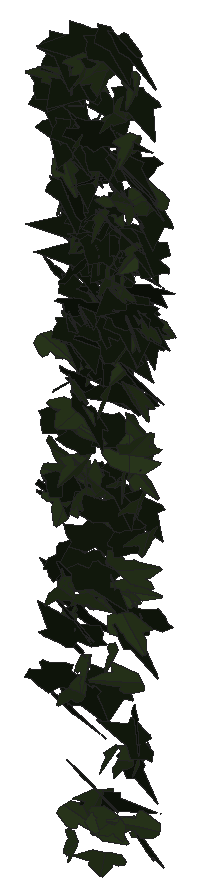
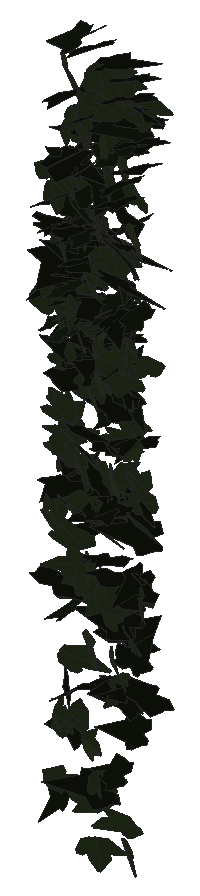
# SketchUp Ruby script. Lengths in millimetres.
U = 1.mm
M = Sketchup.active_model
def pt(a) = Geom::Point3d.new(a.map { |v| v * U })
def face(e, loops, mat)
  f = e.add_face(loops[0].map { |a| pt(a) })
  loops[1..].each { |l| e.add_face(l.map { |a| pt(a) }).erase! }
  f.material = f.back_material = mat if mat
  f
end
# faces: each face lists its corners as indices into pts; further lists are holes
def faces(e, pts, list, mat = nil) = list.each { |f| face(e, (f[0].is_a?(Array) ? f : [f]).map { |l| l.map { |i| pts[i] } }, mat) }
# xy, xz, yz: faces in a plane at the given z, y or x. An outline is a flat list of corners, or four numbers for a rectangle; further outlines are holes
def ring(l) = l.size == 4 ? [[l[0], l[1]], [l[2], l[1]], [l[2], l[3]], [l[0], l[3]]] : l.each_slice(2).to_a
def flat(e, list, mat, &to3) = list.each { |f| face(e, (f[0].is_a?(Array) ? f : [f]).map { |l| ring(l).map { |u, v| to3.(u, v) } }, mat) }
def xy(e, z, list, mat = nil) = flat(e, list, mat) { |x, y| [x, y, z] }
def xz(e, y, list, mat = nil) = flat(e, list, mat) { |x, z| [x, y, z] }
def yz(e, x, list, mat = nil) = flat(e, list, mat) { |y, z| [x, y, z] }
def lines(e, pts, list) = list.each { |a, b| e.add_line(pt(pts[a]), pt(pts[b])) }
# prism: a flat outline (further loops are holes) pulled along v
def prism(e, loops, v, mat = nil)
  f = face(e, loops, mat); d = Geom::Vector3d.new(v.map { |x| x * U })
  f.pushpull(f.normal.samedirection?(d) ? d.length : -d.length)
end
def box(e, o, s, mat = nil) = prism(e, [[o, [o[0] + s[0], o[1], o[2]], [o[0] + s[0], o[1] + s[1], o[2]], [o[0], o[1] + s[1], o[2]]]], [0, 0, s[2]], mat)
def at(x, y, z, deg = 0) = Geom::Transformation.translation(pt([x, y, z])) * Geom::Transformation.rotation(ORIGIN, Z_AXIS, deg.degrees)
def axes(o, x, y, z) = Geom::Transformation.new([*x, 0, *y, 0, *z, 0, *pt(o).to_a, 1])
def part(name) = M.definitions.add(name)
# library, detail: a bought-in or finely detailed component or shape, given as its bounding box
def library(name, o, s) = part(name).tap { |d| box(d.entities, o, s) }
def detail(e, o, s) = box(e.add_group.entities, o, s)
def put(e, d, t, mat = nil) = e.add_instance(d, t).tap { |i| i.material = mat if mat }
def group(e, t, mat = nil) = e.add_group.tap { |g| g.transformation = t; g.material = mat if mat }.entities
root = M.entities
M.materials.add("efeu1").color = [18, 25, 13]
M.materials.add("efeu2").color = [43, 57, 29]
c1 = part("ivyleaf_9")
p = [[39.1,54.8,31.7],[34.5,51.8,30.2],[-5.3,25.2,17.3],[-17.9,28.3,20.9],[-21.6,21.7,17],[-20.2,4.3,5.3],
  [-22.9,-0.3,2.5],[-17.1,-4,-0.6],[-2,-2.1,-1.2],[-0.7,-15.4,-10.1],[16.6,-22.3,-16.7],[21.1,-15.1,-12.5],
  [32.7,-10.7,-11],[46.1,-1.8,-6.6],[30.8,11.2,3.8]]
faces(c1.entities,p,[[0,1,2,3,4,5,6,7,8,9,10,11,12,13,14]],"efeu1")
c2 = part("ivyleaf_10")
p = [[0,12.8,-0.8],[-1.5,51.3,-10.9],[-4.9,51,-11.6],[-13.6,26.5,-7.3],[-13.2,15.9,-4.6],[-21.1,19.3,-7.2],
  [-29.5,16.3,-8.3],[-29.2,8.3,-6.2],[-19.7,-9.8,0.5],[-7.6,-13,4],[1,-12.2,5.8],[-0.4,51.1,-11.1],
  [-1.5,51.1,-10.9],[1,-12.4,5.9],[16.9,-12.4,3.5],[35.1,9.1,-5.1],[35,12.9,-6.1],[20.5,16.4,-4.9],
  [15.8,15,-3.8],[15.3,27.6,-7.1],[12.8,31.3,-7.8]]
faces(c2.entities,p,[[0,1,2,3,4,5,6,7,8,9,10],[11,12,0,13,14,15,16,17,18,19,20]],"efeu2")
put(root,c1,axes([2108.3,967.1,644.8],[1.00488,-0.20839,-0.71065],[1.27223,-0.24155,0.56748],[-0.60667,-0.85174,0.01293]))
put(root,c2,axes([2115.5,961.4,1563.5],[-0.34583,0.64404,-0.48709],[0.15743,-0.4818,-0.6679],[-1.52874,-0.19531,0.04141]))
put(root,c2,axes([2112.9,945,696],[-0.29657,-0.59672,-0.59249],[0.40636,0.55475,-0.61487],[1.54797,-0.25996,0.0479]))
put(root,c2,axes([2130.7,968.5,900.1],[-0.13701,-0.55796,0.633],[0.07222,-0.63679,-0.55699],[1.6043,-0.01898,0.07913]))
put(root,c1,axes([2165,954.3,739.4],[0.05238,-0.56762,-0.51326],[0.37061,0.50188,-0.54459],[1.4085,-0.11095,0.16239]))
put(root,c2,axes([2176.4,947.7,1276],[0.79385,-0.52482,-0.47962],[-0.14077,0.52102,-0.63445],[1.34577,0.36409,0.21656]))
put(root,c1,axes([2140.5,961.2,1130.8],[-0.37396,-0.7341,-0.27689],[0.2109,0.25662,-0.75898],[1.47825,-0.22232,0.03824]))
put(root,c1,axes([2131.3,969.4,1536.4],[-1.26194,-0.47663,0.15068],[-0.01345,-0.24134,-0.7945],[0.95127,-0.6357,0.18866]))
put(root,c2,axes([2101.8,955.2,1545.3],[-1.15192,-0.56127,0.00643],[-0.00965,-0.00399,-0.82544],[1.06823,-0.60528,-0.00052]))
put(root,c1,axes([2146,969.2,995.5],[0.23611,-0.7653,0.36632],[0.0902,-0.36339,-0.77522],[1.61226,0.13241,-0.01027]))
put(root,c1,axes([2132.3,959.9,611.1],[0.74877,0.01244,0.76483],[-1.44263,0.12186,0.38793],[-0.19554,-0.85142,0.06669]))
put(root,c1,axes([2206.7,969.2,886.7],[0.10131,-0.80719,0.28495],[0.02782,-0.2846,-0.80894],[1.62892,0.05506,-0.00391]))
put(root,c1,axes([2158.5,952,1181.7],[0.48377,0.56591,-0.44058],[-0.55888,-0.34433,-0.6117],[-1.2453,0.37437,0.10337]))
put(root,c2,axes([2216.6,949.5,1442.1],[0.30113,-0.68342,-0.44499],[-0.00794,0.4526,-0.6966],[1.55208,0.13491,0.08277]))
put(root,c2,axes([2106.2,963.3,1390.3],[0.94252,-0.3055,0.55505],[0.96578,-0.23056,-0.57966],[0.72199,0.70723,0.05079]))
put(root,c1,axes([2201.5,949.6,838.4],[-0.80201,-0.07863,0.75132],[1.42849,0.05368,0.4266],[-0.16255,0.85975,0.04208]))
put(root,c2,axes([2133.2,957.9,993.3],[1.43151,-0.13805,-0.25891],[-0.48275,0.0522,-0.7647],[0.28072,0.79376,0.00526]))
put(root,c2,axes([2214.5,944.6,1521.6],[-0.1793,-0.63096,-0.69188],[0.24221,0.68029,-0.63772],[1.76559,-0.1574,0.01722]))
put(root,c2,axes([2199.9,956.8,337.1],[1.22763,-0.3477,-0.28676],[-0.47961,0.13685,-0.73278],[0.71115,0.69251,0.00083]))
put(root,c2,axes([2151.9,963.7,1580.9],[-0.42301,-0.77281,0.28209],[0.02369,-0.29533,-0.79928],[1.56556,-0.20434,0.08831]))
put(root,c2,axes([2241.9,957.1,1149],[-0.98131,0.58056,0.05581],[0.07125,-0.0414,0.77647],[1.10772,0.51697,-0.0005]))
put(root,c2,axes([2200.9,944.9,1242.9],[-0.00609,-0.47373,-0.67238],[0.22749,0.66498,-0.46909],[1.54878,-0.09954,0.06626]))
put(root,c2,axes([2185.2,958,1570.4],[-0.35991,-0.81721,-0.02621],[0.03658,0.02245,-0.8387],[1.55569,-0.18959,0.01365]))
put(root,c1,axes([2180.2,954.1,1292.9],[0.33246,-0.61743,-0.53459],[-0.09089,0.53802,-0.637],[1.55169,0.1638,0.07722]))
put(root,c1,axes([2112.2,971.4,1096.9],[0.13468,-0.61448,0.47429],[0.03698,-0.4747,-0.61791],[1.47686,0.06792,-0.02778]))
put(root,c2,axes([2248.2,955.5,882.7],[-0.14702,-0.77871,-0.18603],[0.06326,0.18361,-0.7824],[1.52243,-0.08283,0.01455]))
put(root,c1,axes([2202.5,968.2,1631.3],[-0.00601,-0.84491,0.07539],[0.02466,-0.07543,-0.84481],[1.61423,-0.00199,0.01319]))
put(root,c1,axes([2155.7,947.7,1472.1],[0.42782,0.1624,-0.82068],[0.84608,0.69669,0.25963],[1.34881,-0.48853,0.09744]))
put(root,c1,axes([2156.5,971.5,1599.2],[-0.80069,-0.22964,0.69068],[-1.09651,-0.38244,-0.47809],[0.84652,-0.71259,0.03401]))
put(root,c2,axes([2176.3,968.6,1325.1],[0.19626,-0.60012,0.49082],[0.28629,-0.47025,-0.60657],[1.44747,0.17438,0.05342]))
put(root,c1,axes([2249,969.3,477.5],[-0.11424,-0.7725,-0.20296],[-0.03145,-0.20228,0.77483],[-1.51978,0.06226,-0.00078]))
put(root,c2,axes([2242.8,969.1,1287.6],[0.36474,0.41415,-0.66507],[-0.48325,-0.61489,-0.45607],[-1.41064,0.31773,-0.01572]))
put(root,c2,axes([2141,963.9,1449.9],[0.39218,-0.76636,0.15382],[0.08859,-0.14676,-0.79355],[1.48499,0.21115,0.00672]))
put(root,c2,axes([2222.1,961.5,671.4],[1.26495,-0.04026,0.50054],[0.9502,-0.036,-0.66585],[0.1024,0.83126,-0.00459]))
put(root,c2,axes([2242.8,958.6,963.3],[-0.69401,-0.64345,0.18972],[0.20244,0.15775,0.73945],[-1.26058,0.37958,0.0143]))
put(root,c2,axes([2228.4,970.1,1468.3],[-0.15732,-0.6876,0.47749],[0.23372,-0.48458,-0.67655],[1.576,0.00323,0.148]))
put(root,c1,axes([2118.1,969.4,1587.2],[-0.60978,-0.76889,-0.04698],[0.01297,0.04805,-0.83289],[1.46602,-0.32024,-0.01217]))
put(root,c1,axes([2131,966.2,1454.7],[-0.29413,-0.77185,-0.17177],[0.03353,0.17161,-0.78701],[1.50455,-0.15472,-0.01604]))
put(root,c1,axes([2188.5,964.4,1617.8],[0.05976,-0.81112,-0.24453],[0.18389,0.24653,-0.80535],[1.60183,0.00196,0.10158]))
put(root,c2,axes([2088.1,950.3,1097.4],[0.62224,0.47097,0.47558],[0.33077,0.4514,-0.5665],[-1.23016,0.3596,0.08824]))
put(root,c2,axes([2228.1,945.5,451.7],[-0.16121,-0.41304,-0.77746],[0.434,0.7441,-0.42016],[1.61833,-0.24069,0.03523]))
put(root,c1,axes([2216,957.2,1133.6],[0.02431,-0.53743,-0.54965],[0.16101,0.54737,-0.53324],[1.45417,-0.05162,0.06823]))
put(root,c1,axes([2174,953.4,785.6],[-1.03834,-0.27228,0.60432],[1.06791,0.22693,0.60881],[-0.67153,0.7819,0.03375]))
put(root,c1,axes([2221.9,943.3,1261.9],[0.36594,0.31084,0.71561],[0.3777,0.6933,-0.35447],[-1.43605,0.26155,0.08912]))
put(root,c2,axes([2211.1,972,904.1],[0.3976,-0.4049,0.58719],[0.64532,-0.48192,-0.45295],[1.19428,0.3952,0.04926]))
put(root,c2,axes([2140.3,972.1,571.5],[0.74936,-0.49896,0.51455],[0.56196,-0.42203,-0.63518],[1.24297,0.49161,-0.02304]))
put(root,c1,axes([2192.9,973.1,1310.3],[0.19037,-0.47425,0.62662],[0.65608,-0.54118,-0.46461],[1.34406,0.33134,0.13804]))
put(root,c2,axes([2203.8,959,893.3],[-0.3033,-0.75624,-0.21444],[0.07978,0.21031,-0.77285],[1.4939,-0.16477,-0.00227]))
put(root,c1,axes([2106.5,974.8,1338.9],[-0.06029,-0.79066,0.24981],[0.06375,-0.25101,-0.7902],[1.57681,-0.02008,0.0415]))
put(root,c1,axes([2123.5,968.9,1537.6],[-1.48661,-0.17497,-0.20759],[0.38867,0.03799,-0.80043],[0.34048,-0.80733,0.00732]))
put(root,c1,axes([2202,973.2,1274.4],[-1.09359,-0.53973,0.10431],[-0.14937,-0.06881,-0.78833],[1.03551,-0.57993,-0.00355]))
put(root,c1,axes([2170.6,964.6,1430.4],[0.44508,-0.7372,-0.23846],[-0.13797,0.22717,-0.77341],[1.46814,0.24484,-0.00039]))
put(root,c1,axes([2179,967.9,1291.9],[-1.24505,0.00995,-0.3998],[0.75949,-0.03418,-0.65382],[-0.05008,-0.76592,0.02398]))
put(root,c2,axes([2198.5,959.2,1223.6],[-1.36995,0.23872,-0.05263],[0.10008,-0.00863,-0.75832],[-0.45434,-0.72168,-0.00835]))
put(root,c1,axes([2097.3,963.3,1524.2],[-0.21024,-0.63485,-0.51519],[0.41876,0.47761,-0.63572],[1.49864,-0.22252,0.10536]))
put(root,c1,axes([2107.5,975.9,1438.6],[-0.63133,-0.70773,0.18093],[-0.0499,-0.18705,-0.77973],[1.38938,-0.32831,0.05421]))
put(root,c1,axes([2168.5,955.8,1118.4],[0.97208,0.5818,-0.35925],[-0.4458,-0.27241,-0.77418],[-1.22262,0.5619,-0.00335]))
put(root,c2,axes([2133,951.5,533.2],[-0.48702,-0.55271,-0.66852],[0.58172,0.59484,-0.60879],[1.54498,-0.3982,0.01849]))
put(root,c1,axes([2116.5,947.5,1498.6],[1.23753,0.20008,0.46236],[0.51807,0.4957,-0.59732],[-0.80681,0.62519,0.32564]))
put(root,c1,axes([2095.1,972.7,1487.1],[-0.55034,-0.75904,-0.0645],[0.03749,0.06152,-0.81225],[1.44933,-0.28981,-0.00348]))
put(root,c2,axes([2217.1,974.3,1091.5],[-0.22418,-0.48616,0.52364],[0.03457,-0.53257,-0.49037],[1.35944,-0.06663,0.09882]))
put(root,c1,axes([2206.9,972.5,1081.3],[0.68532,-0.49306,0.55085],[0.60482,-0.44998,-0.61051],[1.27038,0.48022,-0.0065]))
put(root,c1,axes([2229.6,971.8,1166.5],[-0.42622,-0.75531,-0.10656],[0.06153,0.10156,-0.78781],[1.45044,-0.22626,0.00211]))
put(root,c2,axes([2221.5,962.3,1130.5],[0.40902,-0.84956,-0.22005],[-0.13039,0.20962,-0.8762],[1.66515,0.2251,-0.01456]))
put(root,c2,axes([2167.6,958.7,1407.4],[0.73671,-0.6086,-0.35473],[-0.06853,0.38713,-0.70349],[1.33892,0.35468,0.15918]))
put(root,c2,axes([2220.5,963.6,754.2],[-1.10821,-0.11113,0.63829],[1.18772,0.13437,0.59271],[-0.3313,0.85347,-0.01021]))
put(root,c2,axes([2256.1,972.4,334.9],[0.10701,0.03281,0.71911],[-0.93285,-0.52652,0.06235],[1.00339,-0.49301,-0.01873]))
put(root,c1,axes([2209.6,971.3,1626.1],[0.74044,-0.74168,0.11189],[0.10112,-0.09848,-0.83753],[1.42396,0.39266,0.0013]))
put(root,c1,axes([2135.8,948.5,1224.8],[0.06435,0.58839,0.52367],[0.06678,0.52251,-0.58935],[-1.49762,0.04858,-0.00378]))
put(root,c2,axes([2147.4,969.4,834],[-0.9677,-0.52162,-0.13871],[-0.16008,-0.11166,0.72823],[-1.0147,0.51507,0.01739]))
put(root,c1,axes([2222.2,976.4,1214.7],[-1.14279,-0.45341,0.18636],[-0.26257,-0.12647,-0.75222],[0.89526,-0.61586,0.01727]))
put(root,c2,axes([2227.6,955.1,1371.2],[0.70066,-0.28862,-0.66391],[-0.60366,0.60522,-0.43899],[1.2385,0.45828,0.16163]))
put(root,c1,axes([2133,954.3,1323.6],[0.09455,-0.09958,0.80488],[-0.33687,0.78562,0.10812],[-1.50632,-0.18194,0.02634]))
put(root,c1,axes([2221.8,971.5,438.1],[-0.13417,-0.00203,-0.79199],[1.50455,-0.04845,-0.07024],[-0.0915,-0.79365,0.00631]))
put(root,c2,axes([2166.6,968.2,1574.2],[-1.00626,-0.61792,0.22347],[-0.27255,-0.17157,-0.81324],[1.2205,-0.54777,0.00264]))
put(root,c1,axes([2127.9,971.3,385.3],[0.86524,-0.57454,0.27098],[0.32234,-0.21153,-0.73265],[1.16522,0.48515,0.00146]))
put(root,c1,axes([2098.5,970.9,868.3],[-0.87105,0.04819,-0.63271],[1.20412,-0.0251,-0.45957],[-0.0925,-0.78049,-0.02429]))
put(root,c2,axes([2168.8,968.4,363.4],[-0.54747,-0.75884,0.09762],[-0.04577,-0.09528,-0.81145],[1.4554,-0.28844,0.01121]))
put(root,c2,axes([2241.3,980.6,451.5],[0.27481,-0.28787,0.75953],[0.54399,-0.70408,-0.3212],[1.447,0.31937,-0.0235]))
put(root,c2,axes([2135.4,960.4,1171.4],[-0.72105,0.63679,0.1376],[-0.15409,0.11192,-0.74087],[-1.2303,-0.38722,0.01215]))
put(root,c2,axes([2232.5,979.9,1141.7],[-0.29592,-0.04822,0.75409],[0.64808,-0.69175,0.02598],[1.2838,0.33809,0.1607]))
put(root,c1,axes([2128,959.3,1040.9],[-0.25319,0.74721,-0.05839],[0.02385,-0.05708,-0.75896],[-1.42622,-0.1336,-0.00233]))
put(root,c2,axes([2229.2,961.4,935.2],[1.28768,0.4743,-0.08218],[0.09631,0.0709,0.82577],[0.91106,-0.67786,0.02887]))
put(root,c1,axes([2090.5,971.6,699.8],[0.43507,-0.2623,0.67593],[1.02087,-0.41565,-0.34271],[0.9284,0.57998,0.06009]))
put(root,c1,axes([2171.1,970.9,1311.3],[-1.05464,0.35619,-0.41437],[0.6364,-0.2457,-0.65838],[-0.82248,-0.64684,0.02191]))
put(root,c2,axes([2228.9,974.2,1567],[0.91147,-0.66988,0.24731],[0.27692,-0.19999,-0.82347],[1.33052,0.50052,0.00196]))
put(root,c2,axes([2116.6,967,964.2],[-0.65303,-0.10859,-0.60991],[1.1783,-0.08462,-0.33324],[-0.04144,-0.69466,0.13594]))
put(root,c1,axes([2097.8,967.2,969.5],[0.01212,-0.64745,-0.45045],[-0.05376,0.44999,-0.64719],[1.50016,0.02136,-0.01956]))
put(root,c1,axes([2225.8,977.9,511],[-0.2098,0.03209,-0.77064],[1.29403,-0.36351,-0.11239],[-0.69309,-0.6884,0.02343]))
put(root,c1,axes([2189.4,970.1,1060.1],[0.54301,-0.06019,0.74043],[-1.34651,0.21983,0.29049],[-0.4311,-0.76244,0.02531]))
put(root,c2,axes([2083.7,974.2,898.9],[-0.51366,0.01283,0.68452],[1.21982,-0.25394,0.25747],[0.45808,0.69059,0.08196]))
put(root,c2,axes([2218.4,966.2,1168.3],[-0.80693,0.08487,-0.70567],[-1.29819,0.18232,0.43176],[0.38013,0.8028,-0.02346]))
put(root,c2,axes([2200.5,965.8,707.6],[-1.29888,-0.2581,-0.08969],[0.15794,0.03413,-0.72964],[0.49546,-0.68749,-0.00255]))
put(root,c2,axes([2205.8,962,1279.7],[0.26952,-0.62822,-0.41581],[-0.07698,0.41614,-0.6425],[1.43174,0.14064,0.04373]))
put(root,c1,axes([2222.3,974,1407.7],[0.80845,-0.67911,0.09071],[0.06213,-0.08655,-0.80082],[1.30248,0.42565,-0.0181]))
put(root,c2,axes([2125.7,962.5,1033.4],[-0.99469,0.53881,0.21262],[-0.3275,0.12902,-0.74994],[-1.05264,-0.54928,0.03241]))
put(root,c2,axes([2231.1,966.7,1055.2],[-1.27775,0.44723,-0.17969],[0.28505,-0.09927,-0.80669],[-0.87188,-0.68787,-0.0004]))
put(root,c1,axes([2129.8,976.7,1191.3],[-0.08795,-0.78724,-0.05396],[0.02741,0.05321,-0.78851],[1.50153,-0.04708,0.01123]))
put(root,c2,axes([2098.7,972.5,828.6],[1.37804,-0.4739,0.08186],[0.12642,-0.04799,-0.86535],[0.90651,0.7271,-0.00376]))
put(root,c1,axes([2143,973.5,1290.3],[-1.17918,0.04282,0.46131],[-0.87854,0.00845,-0.62077],[-0.07498,-0.77241,0.01878]))
put(root,c1,axes([2108.6,974.4,1560.2],[-0.33294,-0.77201,-0.2741],[0.12381,0.2663,-0.79157],[1.55423,-0.18659,0.00434]))
put(root,c1,axes([2231.1,958.5,1190.1],[-0.03374,-0.07388,-0.76761],[0.32531,0.74834,-0.07597],[1.43116,-0.17184,-0.00083]))
put(root,c1,axes([2207.7,979.9,1414.6],[0.46524,-0.62224,0.46266],[0.44838,-0.40257,-0.6659],[1.40596,0.33429,0.05927]))
put(root,c1,axes([2121.3,973.5,524.9],[-0.18943,-0.1287,-0.80002],[1.50011,0.17158,-0.12567],[0.3577,-0.78772,0.10334]))
put(root,c2,axes([2178.1,979.2,1035.4],[0.45758,-0.75117,0.41228],[0.2921,-0.38353,-0.78829],[1.60443,0.28406,0.02593]))
put(root,c2,axes([2180.1,960.9,310.9],[0.82222,0.20004,-0.62224],[1.02708,0.31162,0.47487],[0.70177,-0.69045,0.03404]))
put(root,c2,axes([2200.4,976.1,821.2],[-0.76024,-0.12453,-0.69293],[-1.25633,-0.21074,0.41841],[-0.46584,0.77156,0.00244]))
put(root,c1,axes([2270.2,973.2,1286.4],[-1.21547,0.09547,0.5697],[-1.0682,0.09821,-0.64566],[-0.25989,-0.85016,-0.01062]))
put(root,c1,axes([2215.4,973.7,647.9],[0.70014,-0.7401,-0.13066],[-0.11158,0.11677,-0.82649],[1.42598,0.37252,-0.00052]))
put(root,c2,axes([2199.1,971,1232.1],[0.90937,-0.59829,-0.11606],[-0.11242,0.10131,-0.76548],[1.15442,0.48115,0.01688]))
put(root,c2,axes([2104.1,960.6,705.7],[0.3977,-0.41407,-0.59617],[-0.28329,0.58276,-0.45692],[1.3521,0.24389,0.07962]))
put(root,c2,axes([2121.9,964.6,1292.1],[0.65248,-0.596,-0.44686],[-0.28634,0.42638,-0.6841],[1.3885,0.368,0.06891]))
put(root,c2,axes([2232.9,981.2,448.1],[-0.29654,-0.49359,0.55589],[-0.25051,-0.54068,-0.51698],[1.39249,-0.20238,0.02538]))
put(root,c1,axes([2073.9,961.8,537.8],[0.28551,0.02576,-0.76784],[0.6995,0.6846,0.09478],[1.284,-0.37869,0.1191]))
put(root,c2,axes([2172.7,960.9,884.4],[-0.07236,0.07536,0.85124],[-1.4561,0.3766,-0.06751],[-0.72456,-0.76435,0.05066]))
put(root,c2,axes([2108.9,976.7,632.1],[0.87066,-0.57077,0.20846],[0.2431,-0.16478,-0.73147],[1.13064,0.47496,-0.00325]))
put(root,c1,axes([2161.6,955.9,1385.6],[0.60934,0.68552,0.29584],[0.13255,0.29307,-0.75447],[-1.4148,0.3227,0.05673]))
put(root,c1,axes([2113.4,975.8,647.8],[0.86111,-0.37743,0.57126],[0.91235,-0.31426,-0.58731],[0.93039,0.65749,0.04721]))
put(root,c2,axes([2253.9,971.2,821.1],[-0.37288,-0.8263,-0.09777],[0.06693,0.09213,-0.84912],[1.58218,-0.19864,0.01288]))
put(root,c1,axes([2254.1,974.2,669.5],[0.2428,-0.05148,0.74925],[-1.36885,0.21037,0.13692],[-0.41141,-0.73034,-0.01337]))
put(root,c1,axes([2209.4,970.9,1431],[0.56983,-0.65219,-0.36735],[-0.09875,0.37661,-0.71093],[1.42118,0.28767,0.09789]))
put(root,c1,axes([2229.2,966.9,808.7],[-1.11382,0.50797,0.40518],[-0.62773,0.23759,-0.77426],[-1.06549,-0.67099,0.03259]))
put(root,c2,axes([2249.8,968.3,1171.1],[-1.24484,0.26856,0.21992],[-0.42331,0.03592,-0.70537],[-0.50719,-0.68912,0.04894]))
put(root,c2,axes([2219,979.2,563.5],[-0.35657,-0.13027,0.72521],[-1.06907,-0.45899,-0.22757],[0.90749,-0.5919,0.01686]))
put(root,c2,axes([2131.5,975.5,1576.9],[-0.79055,-0.68563,0.16225],[-0.11079,-0.1543,-0.8011],[1.33634,-0.4184,0.02957]))
put(root,c2,axes([2129.2,957.8,1126.1],[-0.13939,0.12878,-0.83192],[-0.61156,0.76756,0.14711],[1.48086,0.32911,-0.01755]))
put(root,c1,axes([2224.2,978.1,1048.4],[0.01259,0.04927,-0.80859],[-0.94747,-0.63767,-0.04293],[-1.21629,0.49724,0.02507]))
put(root,c2,axes([2099.6,972.7,962.2],[-0.77202,0.53869,-0.20779],[0.2642,-0.15551,-0.67413],[-1.06663,-0.42842,-0.01658]))
put(root,c1,axes([2147.7,975.4,1158.8],[0.70588,-0.68105,-0.15357],[-0.14249,0.13409,-0.77549],[1.32105,0.37837,-0.00159]))
put(root,c2,axes([2179.9,983.7,713.2],[-0.4418,0.28947,0.71111],[0.86857,-0.54538,0.37099],[1.17505,0.51197,-0.00686]))
put(root,c1,axes([2151.3,974.5,939.4],[-1.14424,-0.50728,0.05018],[0.17217,-0.02982,0.78246],[-0.95477,0.60257,0.08096]))
put(root,c1,axes([2189.8,966.8,1157.2],[0.53949,-0.52808,-0.61317],[-0.46963,0.56235,-0.59839],[1.46676,0.37429,0.03394]))
put(root,c1,axes([2125.8,978.5,1135.7],[0.34636,-0.75284,-0.09867],[-0.0377,0.09673,-0.77452],[1.44458,0.18303,0.00344]))
put(root,c1,axes([2147.5,983.1,1160.9],[0.21784,-0.73491,0.16893],[0.05535,-0.16643,-0.74377],[1.4341,0.11806,0.00305]))
put(root,c2,axes([2196,973.3,708.8],[-1.04463,0.23511,-0.41374],[0.72733,-0.15857,-0.5971],[-0.53967,-0.66881,-0.00387]))
put(root,c2,axes([2159.7,973.7,700.6],[-1.27484,-0.4833,0.09558],[-0.13253,-0.06682,-0.82588],[0.92822,-0.67332,0.01335]))
put(root,c1,axes([2215.5,971,1183.8],[-0.25458,-0.28432,-0.73592],[0.90126,0.56807,-0.30554],[1.20094,-0.48659,0.0733]))
put(root,c2,axes([2119.1,969.1,264.8],[0.48557,-0.60969,-0.39956],[-0.27355,0.37294,-0.66085],[1.36011,0.29267,0.00973]))
put(root,c2,axes([2152.1,968.9,1270.7],[-0.85584,-0.49073,-0.36968],[0.48129,0.26967,-0.6656],[1.06567,-0.5159,0.00372]))
put(root,c2,axes([2082.1,966.6,868.8],[0.19918,-0.05279,0.69107],[0.96539,0.4821,-0.03999],[-0.89889,0.50607,0.11019]))
put(root,c1,axes([2197.4,982.2,1309.5],[-0.95568,-0.56983,-0.24591],[0.34754,0.16666,-0.75908],[1.12888,-0.53371,0.02551]))
put(root,c1,axes([2168.4,989.4,1158.9],[-0.36141,-0.62733,0.39079],[-0.04202,-0.39849,-0.65041],[1.40601,-0.17316,0.08101]))
put(root,c1,axes([2223.1,984.2,1282.2],[-0.77027,-0.05704,0.74689],[-1.38847,-0.16255,-0.40773],[0.32337,-0.8338,0.02839]))
put(root,c1,axes([2234.4,981.4,1303],[0.00641,-0.78001,-0.14313],[0.02505,0.14317,-0.7799],[1.5091,0.00094,0.01355]))
put(root,c2,axes([2207.7,980.1,1501],[-0.33307,-0.81085,0.17773],[-0.05911,-0.17511,-0.8295],[1.57874,-0.17762,0.00644]))
put(root,c1,axes([2099.7,981.6,589.5],[0.81324,-0.59077,0.26814],[-0.28291,0.22339,0.72904],[-1.2019,-0.45231,0.00983]))
put(root,c1,axes([2236.4,963.9,1229],[1.23568,0.46368,0.09757],[0.14578,0.06063,-0.79782],[-0.88994,0.65375,0.00479]))
put(root,c1,axes([2185.2,981.7,1256],[0.71255,-0.43591,0.54064],[0.8179,-0.33705,-0.56937],[1.03828,0.56467,0.0775]))
put(root,c2,axes([2215.9,983.3,986.2],[0.04316,-0.10955,0.76404],[1.36011,-0.28582,-0.0622],[0.55502,0.70893,0.09299]))
put(root,c2,axes([2270.2,982.5,1166],[-0.40453,-0.15598,0.72531],[-1.11372,-0.42853,-0.26365],[0.86793,-0.62259,-0.00025]))
put(root,c2,axes([2180.1,986.6,430.7],[0.26793,-0.54058,0.47041],[0.19302,-0.45955,-0.55845],[1.3501,0.17298,-0.01351]))
put(root,c1,axes([2176.3,977,1324.2],[-1.32912,0.30086,0.13229],[-0.23837,0.04361,-0.76035],[-0.57831,-0.70944,0.00936]))
put(root,c1,axes([2180.5,986.5,1508.6],[-0.13771,-0.80977,0.03417],[0.0008,-0.03434,-0.81298],[1.54252,-0.07228,0.00347]))
put(root,c2,axes([2223.2,983.6,909.4],[0.37939,-0.06304,0.73639],[1.30714,-0.26595,-0.20869],[0.51962,0.71504,-0.0127]))
put(root,c1,axes([2156.8,984.6,886.7],[-0.13001,-0.10657,-0.76198],[1.45722,-0.08462,-0.05681],[-0.14396,-0.76034,0.11312]))
put(root,c2,axes([2156.5,969.5,689.4],[-0.89976,-0.514,-0.45629],[0.56262,0.34791,-0.69819],[1.18092,-0.55738,-0.01502]))
put(root,c2,axes([2124,989.5,883.4],[0.20084,-0.37867,-0.65909],[0.36399,-0.63077,0.39302],[-1.40012,-0.2183,0.00763]))
put(root,c2,axes([2211.4,964.9,715.8],[0.01241,0.04546,0.77785],[0.71068,0.68255,-0.04302],[-1.30154,0.37313,-0.01607]))
put(root,c2,axes([2188.3,976.3,599.1],[0.47684,-0.72504,-0.19623],[-0.11321,0.18705,-0.76709],[1.42504,0.25747,0.00472]))
put(root,c2,axes([2120.2,971.2,1121],[-1.07846,0.37683,0.32052],[-0.51923,0.16852,-0.68044],[-0.78541,-0.62883,0.00972]))
put(root,c2,axes([2151.1,978.2,1470.7],[-0.03123,-0.81,-0.0689],[0.03522,0.06853,-0.80999],[1.54676,-0.01792,0.01705]))
put(root,c2,axes([2183.2,979.8,1337.9],[1.1963,-0.48335,-0.03124],[-0.02742,0.0325,-0.79274],[0.92143,0.62851,0.01697]))
put(root,c1,axes([2122.6,988.2,1204.1],[0.42304,-0.68125,0.31969],[0.24032,-0.29486,-0.71612],[1.41191,0.25431,0.0261]))
put(root,c2,axes([2154.9,986.2,1070.4],[0.1839,-0.71428,0.33007],[0.11213,-0.32505,-0.72066],[1.49334,0.11237,0.01346]))
put(root,c1,axes([2237.1,973.1,318],[1.07601,-0.36927,-0.42469],[-0.67397,0.23445,-0.67528],[0.83246,0.66712,0.00223]))
put(root,c1,axes([2096.9,962.2,737.5],[0.13848,-0.05628,-0.90504],[-0.76385,0.81218,-0.08277],[1.54756,0.40591,0.04013]))
put(root,c1,axes([2121.5,989.2,1461.6],[0.39736,-0.72157,0.37063],[0.43032,-0.31578,-0.74215],[1.48268,0.28503,0.11607]))
put(root,c1,axes([2111.6,980.8,1027],[0.88639,-0.30649,0.52179],[0.86647,-0.2563,-0.55691],[0.75874,0.65075,0.02641]))
put(root,c1,axes([2110.1,974.9,865.8],[-0.19605,-0.50329,-0.68042],[0.33728,0.65742,-0.5131],[1.57502,-0.20343,0.02518]))
put(root,c1,axes([2152.4,975.7,844.6],[1.40401,-0.27338,-0.072],[-0.12793,0.02583,-0.78674],[0.5226,0.74077,0.00086]))
put(root,c1,axes([2221.5,967.9,921.8],[-1.12914,0.2315,-0.42189],[-0.74121,0.16242,0.6368],[0.53799,0.70964,-0.00812]))
put(root,c1,axes([2076.8,987.1,1193.6],[0.62826,-0.63873,0.28091],[0.29287,-0.23647,-0.71852],[1.29531,0.36327,0.02621]))
put(root,c2,axes([2169.5,979.2,254.7],[-1.07711,-0.51041,0.04357],[-0.06027,-0.02994,-0.76211],[0.97309,-0.56683,0.00102]))
put(root,c1,axes([2193.2,993.5,1351.5],[0.15678,-0.52453,0.64775],[0.37539,-0.62015,-0.52726],[1.54125,0.2044,0.06253]))
put(root,c1,axes([2123.1,988.7,1383.6],[-0.32214,-0.77638,-0.03937],[-0.01152,0.04161,-0.79448],[1.47946,-0.16873,-0.01476]))
put(root,c2,axes([2139.4,979.1,1280.9],[-1.33929,-0.23781,0.16983],[-0.29746,-0.06789,-0.74267],[0.46993,-0.72071,0.01392]))
put(root,c1,axes([2132.9,981.5,1094.4],[0.91269,-0.61319,-0.08546],[-0.07644,0.07706,-0.77828],[1.17581,0.48098,0.01574]))
put(root,c2,axes([2161.4,984.4,1101.5],[0.28472,-0.73188,0.13676],[0.0386,-0.13544,-0.74698],[1.41649,0.1508,-0.00714]))
put(root,c2,axes([2254.9,981.1,1390.4],[-1.23347,0.13698,0.41878],[-0.83856,-0.2064,-0.61436],[0.00554,-0.74351,0.2477]))
put(root,c2,axes([2131.9,993.4,669.9],[0.08013,-0.3302,0.6621],[0.16318,-0.65653,-0.33287],[1.39864,0.09552,0.0009]))
put(root,c1,axes([2154.7,980.5,1181.9],[1.01297,-0.54154,-0.08727],[-0.06459,0.08886,-0.75837],[1.04196,0.53198,0.03783]))
put(root,c1,axes([2128.9,984.7,738],[-0.67276,-0.59308,-0.37565],[0.41619,0.30664,-0.6899],[1.26965,-0.41478,0.0271]))
put(root,c1,axes([2143.4,968.6,1295.2],[-0.35144,0.65837,0.36688],[-0.33964,0.3288,-0.67985],[-1.39363,-0.24616,0.07316]))
put(root,c1,axes([2218,995.5,1122.2],[-0.26821,-0.58061,0.4936],[0.08437,-0.50736,-0.58415],[1.44791,-0.07799,0.12547]))
put(root,c1,axes([2220.1,984.3,1535.1],[0.05247,-0.77223,-0.27105],[-0.00968,0.27104,-0.77271],[1.55759,0.0277,0.00433]))
put(root,c2,axes([2097.5,984.5,1331.9],[0.57331,-0.76115,0.04639],[0.01233,-0.04732,-0.81852],[1.45126,0.30109,-0.01137]))
put(root,c1,axes([2175.3,967.3,1060.9],[-0.15149,-0.05712,0.82665],[1.02492,0.62759,0.09522],[-1.19856,0.54389,-0.02306]))
put(root,c1,axes([2063.9,980.6,822.1],[1.21087,-0.21354,0.49065],[0.87209,-0.17624,-0.67089],[0.52594,0.78387,-0.01718]))
put(root,c2,axes([2230.7,984.9,933.9],[-0.4971,-0.70804,0.14131],[-0.09699,-0.13181,-0.75467],[1.37068,-0.26611,-0.00215]))
put(root,c1,axes([2188.3,992,1261.4],[-0.52552,-0.72698,0.016],[-0.01216,-0.01468,-0.77765],[1.38387,-0.2762,-0.00076]))
put(root,c1,axes([2176.4,988.9,1309.9],[0.7407,-0.65365,0.20644],[0.20333,-0.17665,-0.76074],[1.28866,0.40358,0.00138]))
put(root,c1,axes([2221.3,979.4,860.6],[-0.33461,-0.43034,-0.60026],[0.39807,0.56277,-0.46472],[1.34813,-0.27298,-0.01177]))
put(root,c1,axes([2201.3,986.4,1352.6],[-1.14344,0.40455,-0.30162],[0.29541,-0.29809,-0.70898],[-0.91382,-0.60256,0.14822]))
put(root,c1,axes([2145,983.5,1240.7],[-1.23821,0.20394,0.39045],[-0.72561,0.08812,-0.68131],[-0.41992,-0.75363,0.02599]))
put(root,c1,axes([2162.3,971.3,351.4],[0.35318,0.30961,-0.69755],[0.67242,0.60146,0.36095],[1.28745,-0.39907,0.00284]))
put(root,c2,axes([2244.1,979.2,1282],[0.40745,-0.69798,-0.30106],[-0.18472,0.28512,-0.73003],[1.43486,0.23491,-0.00849]))
put(root,c1,axes([2152.4,979.2,1186.7],[0.5685,0.59046,-0.43472],[-0.31897,-0.402,-0.66118],[-1.35853,0.34147,-0.02668]))
put(root,c2,axes([2110,978.5,309.1],[0.67757,0.15154,0.64477],[1.11584,0.26844,-0.38682],[-0.58644,0.68587,0.00894]))
put(root,c1,axes([2078.6,986.6,481.9],[1.03644,-0.47213,0.31437],[0.45072,-0.20674,-0.72074],[0.98093,0.59384,-0.00099]))
put(root,c2,axes([2150.4,994.8,1137.7],[-0.43957,-0.13339,0.70643],[0.94863,-0.56441,0.05638],[0.986,0.48356,0.26069]))
put(root,c1,axes([2111.5,984.3,1418.4],[0.23018,-0.72043,-0.33191],[-0.01722,0.33448,-0.72929],[1.50955,0.11367,0.04229]))
put(root,c1,axes([2167.3,994.2,540.9],[-0.35853,-0.78177,0.09077],[-0.04117,-0.08816,-0.80415],[1.4973,-0.18962,-0.00037]))
put(root,c2,axes([2191.1,985.5,1154.9],[-1.19277,-0.06817,0.37557],[-0.63466,-0.25357,-0.60248],[0.35351,-0.68522,0.18558]))
put(root,c2,axes([2113.2,981.2,1077.1],[1.1862,0.30802,0.18403],[0.25642,0.14096,-0.69223],[-0.63292,0.6344,0.06446]))
put(root,c1,axes([2228.8,995,1142.4],[0.03252,-0.72583,0.23978],[0.1182,-0.23773,-0.72405],[1.45002,0.03566,0.05365]))
put(root,c2,axes([2136.2,995.5,1106.7],[-0.37374,-0.27838,0.66925],[-0.37475,-0.64681,-0.32682],[1.32763,-0.26094,0.09615]))
put(root,c1,axes([2213.5,996.2,1202.2],[0.02944,-0.69659,0.34377],[0.21071,-0.33835,-0.69059],[1.46332,0.06274,0.09253]))
put(root,c2,axes([2120.4,978.7,1546.9],[-1.16219,-0.2846,-0.48513],[0.86843,0.16799,-0.67291],[0.62585,-0.76159,0.03286]))
put(root,c2,axes([2246.2,985.6,1363.2],[-0.30587,-0.7675,0.0093],[0.10548,-0.02108,-0.78196],[1.457,-0.15959,0.05856]))
put(root,c2,axes([2167.1,984.1,1051.8],[-1.03709,0.40266,-0.30524],[0.46771,-0.18104,-0.67755],[-0.84024,-0.59777,-0.00041]))
put(root,c1,axes([2241,995.3,1349.5],[-0.2644,-0.7766,0.1023],[0.0007,-0.10396,-0.78871],[1.4908,-0.13768,0.01851]))
put(root,c1,axes([2220.8,994.3,1426.4],[-0.14054,0.24379,-0.83335],[-0.07843,-0.8364,-0.24103],[-1.65065,0.01899,0.08241]))
put(root,c1,axes([2194.8,988.6,965.4],[-1.46777,0.07208,0.10213],[-0.19394,0.00721,-0.77457],[-0.1378,-0.77791,0.00229]))
